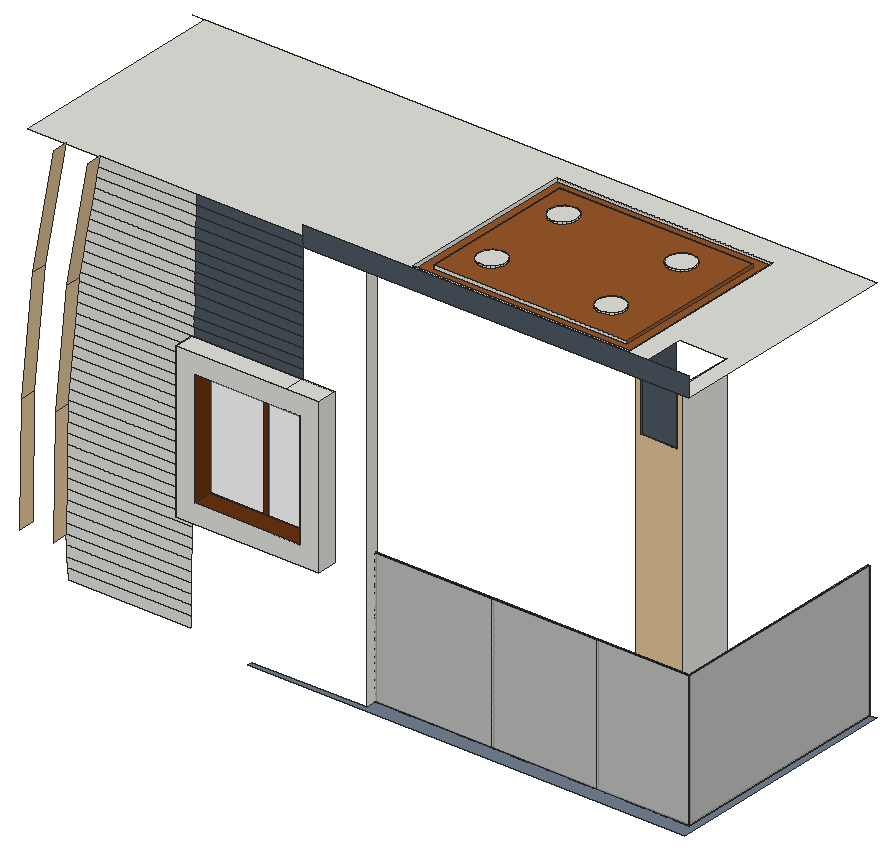
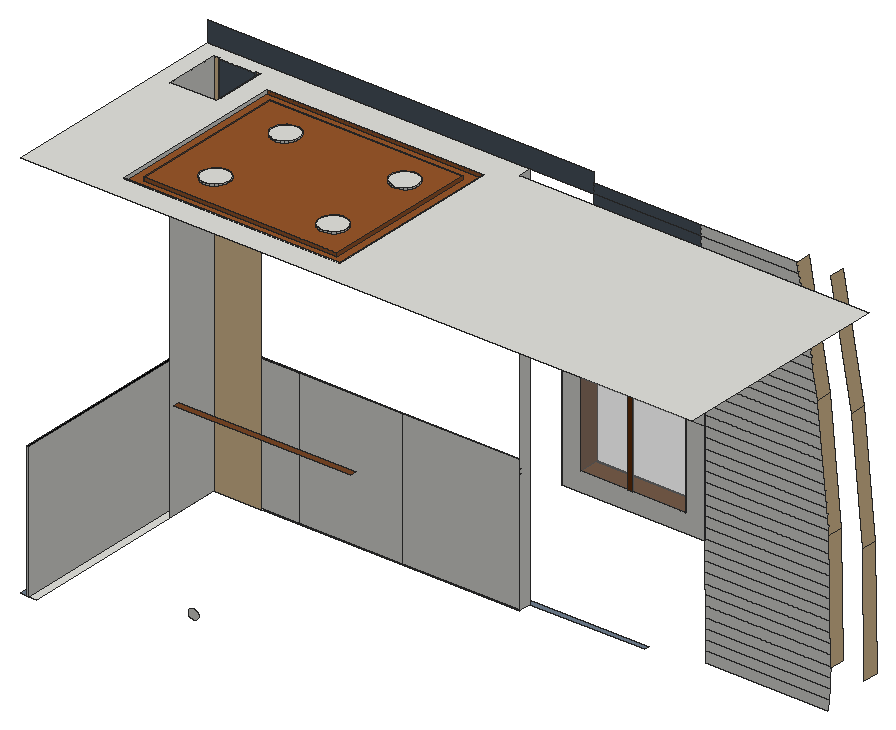
# SketchUp Ruby script. Lengths in inches.
U = 1.inch
M = Sketchup.active_model
def pt(a) = Geom::Point3d.new(a.map { |v| v * U })
def face(e, loops, mat)
  f = e.add_face(loops[0].map { |a| pt(a) })
  loops[1..].each { |l| e.add_face(l.map { |a| pt(a) }).erase! }
  f.material = f.back_material = mat if mat
  f
end
# faces: each face lists its corners as indices into pts; further lists are holes
def faces(e, pts, list, mat = nil) = list.each { |f| face(e, (f[0].is_a?(Array) ? f : [f]).map { |l| l.map { |i| pts[i] } }, mat) }
# xy, xz, yz: faces in a plane at the given z, y or x. An outline is a flat list of corners, or four numbers for a rectangle; further outlines are holes
def ring(l) = l.size == 4 ? [[l[0], l[1]], [l[2], l[1]], [l[2], l[3]], [l[0], l[3]]] : l.each_slice(2).to_a
def flat(e, list, mat, &to3) = list.each { |f| face(e, (f[0].is_a?(Array) ? f : [f]).map { |l| ring(l).map { |u, v| to3.(u, v) } }, mat) }
def xy(e, z, list, mat = nil) = flat(e, list, mat) { |x, y| [x, y, z] }
def xz(e, y, list, mat = nil) = flat(e, list, mat) { |x, z| [x, y, z] }
def yz(e, x, list, mat = nil) = flat(e, list, mat) { |y, z| [x, y, z] }
def lines(e, pts, list) = list.each { |a, b| e.add_line(pt(pts[a]), pt(pts[b])) }
# prism: a flat outline (further loops are holes) pulled along v
def prism(e, loops, v, mat = nil)
  f = face(e, loops, mat); d = Geom::Vector3d.new(v.map { |x| x * U })
  f.pushpull(f.normal.samedirection?(d) ? d.length : -d.length)
end
def box(e, o, s, mat = nil) = prism(e, [[o, [o[0] + s[0], o[1], o[2]], [o[0] + s[0], o[1] + s[1], o[2]], [o[0], o[1] + s[1], o[2]]]], [0, 0, s[2]], mat)
def at(x, y, z, deg = 0) = Geom::Transformation.translation(pt([x, y, z])) * Geom::Transformation.rotation(ORIGIN, Z_AXIS, deg.degrees)
def axes(o, x, y, z) = Geom::Transformation.new([*x, 0, *y, 0, *z, 0, *pt(o).to_a, 1])
def part(name) = M.definitions.add(name)
# library, detail: a bought-in or finely detailed component or shape, given as its bounding box
def library(name, o, s) = part(name).tap { |d| box(d.entities, o, s) }
def detail(e, o, s) = box(e.add_group.entities, o, s)
def put(e, d, t, mat = nil) = e.add_instance(d, t).tap { |i| i.material = mat if mat }
def group(e, t, mat = nil) = e.add_group.tap { |g| g.transformation = t; g.material = mat if mat }.entities
root = M.entities
M.materials.add("[0033_NavajoWhite]").color = [226, 197, 153]
M.materials.add("[0043_SaddleBrown]").color = [104, 51, 14]
M.materials.add("[0111_SlateGray]").color = [77, 88, 99]
M.materials.add("[0111_SlateGray]1").color = [112, 128, 144]
M.materials.add("[0137_Black]").color = [0, 0, 0]
M.materials.add("[Translucent Glass Gray]").color = [193, 193, 193]
M.materials["[Translucent Glass Gray]"].alpha = 0.5
M.materials.add("[Translucent Resin Crush Gray]").color = [184, 184, 184]
M.materials["[Translucent Resin Crush Gray]"].alpha = 0.8
M.materials.add("[Wood Cherry Original]").color = [152, 86, 42]
M.materials.add("[Wood Veneer 01]").color = [120, 70, 37]
xy(root,1006.5625,[[648,136.125,1210.3,139.125],[1210.3,136.125,1212.3,136.125,1212.3,538.125,1208.3,538.125,1208.3,139.125,1210.3,139.125],[648,139.125,1208.3,139.125,1208.3,538.125,1195.125,538.125,1195.125,142.125,648,142.125]])
xy(root,1006.5625,[[444,109.125,1224,109.125,1224,538.125,1212.3,538.125,1212.3,136.125,648,136.125,648,118.125,444,118.125]],"[0111_SlateGray]1")
xy(root,1217.72,[[336.04,82.125,592.16,118.125]])
xy(root,1246.5625,[[648,136.125,858.37,139.125],[858.37,136.125,1045.72,139.125],[1045.72,136.125,1210.3,139.125],[1210.3,136.125,1212.3,136.125,1212.3,538.125,1208.3,538.125,1208.3,139.125,1210.3,139.125]],"[0137_Black]")
xy(root,1251.48,[[369.8,82.125,558.4,118.125]],"[0043_SaddleBrown]")
xy(root,1411.875,[[624,538.125,939.8125,550.125]],"[Wood Veneer 01]")
xy(root,1458.02,[[391.68,95.13,389.33,95.2,387.08,95.88,385.08,97.12,383.47,98.83,382.36,100.9,381.82,103.18,381.89,105.53,382.57,107.78,383.8,109.78,385.51,111.39,387.58,112.5,389.87,113.04,392.22,112.97,394.47,112.29,396.47,111.06,398.08,109.35,399.1875,107.28,399.73,104.99,399.66,102.64,398.98,100.39,397.74,98.39,396.03,96.78,393.96,95.67],[453.68,95.13,451.33,95.2,449.08,95.88,447.08,97.12,445.47,98.83,444.36,100.9,443.82,103.18,443.89,105.53,444.57,107.78,445.8,109.78,447.51,111.39,449.58,112.5,451.87,113.04,454.22,112.97,456.47,112.29,458.47,111.06,460.08,109.35,461.1875,107.28,461.73,104.99,461.66,102.64,460.98,100.39,459.74,98.39,458.03,96.78,455.96,95.67],[516.12,95.13,513.77,95.2,511.52,95.88,509.52,97.12,507.91,98.83,506.8,100.9,506.26,103.18,506.33,105.53,507,107.78,508.24,109.78,509.95,111.39,512.02,112.5,514.31,113.04,516.66,112.97,518.91,112.29,520.9,111.06,522.51,109.35,523.625,107.28,524.17,104.99,524.09,102.64,523.42,100.39,522.18,98.39,520.47,96.78,518.4,95.67]])
xy(root,1458.02,[[[369.8,82.125,558.4,118.125],[391.68,95.13,393.96,95.67,396.03,96.78,397.74,98.39,398.98,100.39,399.66,102.64,399.73,104.99,399.1875,107.28,398.08,109.35,396.47,111.06,394.47,112.29,392.22,112.97,389.87,113.04,387.58,112.5,385.51,111.39,383.8,109.78,382.57,107.78,381.89,105.53,381.82,103.18,382.36,100.9,383.47,98.83,385.08,97.12,387.08,95.88,389.33,95.2],[453.68,95.13,455.96,95.67,458.03,96.78,459.74,98.39,460.98,100.39,461.66,102.64,461.73,104.99,461.1875,107.28,460.08,109.35,458.47,111.06,456.47,112.29,454.22,112.97,451.87,113.04,449.58,112.5,447.51,111.39,445.8,109.78,444.57,107.78,443.89,105.53,443.82,103.18,444.36,100.9,445.47,98.83,447.08,97.12,449.08,95.88,451.33,95.2],[516.12,95.13,518.4,95.67,520.47,96.78,522.18,98.39,523.42,100.39,524.09,102.64,524.17,104.99,523.625,107.28,522.51,109.35,520.9,111.06,518.91,112.29,516.66,112.97,514.31,113.04,512.02,112.5,509.95,111.39,508.24,109.78,507,107.78,506.33,105.53,506.26,103.18,506.8,100.9,507.91,98.83,509.52,97.12,511.52,95.88,513.77,95.2]]],"[0043_SaddleBrown]")
xy(root,1491.78,[[336.04,82.125,534.32,118.125],[534.32,82.125,592.16,118.125]])
xy(root,1596.63,[[1110.4375,146.89,1112.4375,229.71]],"[0111_SlateGray]")
xy(root,1598.625,[[1119.45,142.125,1184.58,144.125]],"[0111_SlateGray]")
xy(root,1698,[[[688.77,171.82,1075.45,493.51],[709.36,192.42,1054.86,472.91]]],"[Wood Cherry Original]")
xy(root,1704,[[[648,118.125,648,142.125,24,142.125,24,538.125,1224,538.125,1224,118.125],[688.77,171.82,1075.45,493.51],[1110.4375,142.125,1119.45,142.125,1119.45,144.125,1184.58,144.125,1184.58,142.125,1195.125,142.125,1195.125,239.75,1110.4375,239.75,1110.4375,229.71,1112.4375,229.71,1112.4375,146.89,1110.4375,146.89]]])
xy(root,1704,[[[709.36,192.42,1054.86,472.91],[765.56,231.1,771.66,232.53,777.18,235.49,781.75,239.78,785.05,245.1,786.86,251.1,787.0625,257.36,785.63,263.46,782.67,268.99,778.39,273.55,773.0625,276.86,767.0625,278.67,760.8,278.87,754.7,277.4375,749.18,274.48,744.61,270.19,741.31,264.87,739.5,258.87,739.3,252.61,740.73,246.51,743.6875,240.99,747.97,236.42,753.3,233.11,759.29,231.3],[978.37,231.1,984.47,232.53,989.99,235.49,994.56,239.78,997.86,245.1,999.68,251.1,999.875,257.36,998.44,263.46,995.49,268.99,991.2,273.55,985.875,276.86,979.875,278.67,973.61,278.87,967.51,277.4375,961.99,274.48,957.42,270.19,954.12,264.87,952.31,258.87,952.11,252.61,953.54,246.51,956.5,240.99,960.79,236.42,966.11,233.11,972.11,231.3],[978.37,388.48,984.47,389.91,989.99,392.87,994.56,397.15,997.86,402.48,999.68,408.48,999.875,414.74,998.44,420.84,995.49,426.36,991.2,430.93,985.875,434.23,979.875,436.04,973.61,436.24,967.51,434.8125,961.99,431.85,957.42,427.57,954.12,422.24,952.31,416.25,952.11,409.98,953.54,403.88,956.5,398.36,960.79,393.79,966.11,390.49,972.11,388.68],[765.56,391.23,771.66,392.66,777.18,395.62,781.75,399.9,785.05,405.23,786.86,411.23,787.0625,417.49,785.63,423.59,782.67,429.11,778.39,433.68,773.0625,436.98,767.0625,438.79,760.8,438.99,754.7,437.5625,749.18,434.6,744.61,430.32,741.31,424.99,739.5,419,739.3,412.73,740.73,406.63,743.6875,401.11,747.97,396.54,753.3,393.24,759.29,391.43]]],"[Wood Cherry Original]")
xy(root,1707,[[765.56,231.1,759.29,231.3,753.3,233.11,747.97,236.42,743.6875,240.99,740.73,246.51,739.3,252.61,739.5,258.87,741.31,264.87,744.61,270.19,749.18,274.48,754.7,277.4375,760.8,278.87,767.0625,278.67,773.0625,276.86,778.39,273.55,782.67,268.99,785.63,263.46,787.0625,257.36,786.86,251.1,785.05,245.1,781.75,239.78,777.18,235.49,771.66,232.53],[978.37,231.1,972.11,231.3,966.11,233.11,960.79,236.42,956.5,240.99,953.54,246.51,952.11,252.61,952.31,258.87,954.12,264.87,957.42,270.19,961.99,274.48,967.51,277.4375,973.61,278.87,979.875,278.67,985.875,276.86,991.2,273.55,995.49,268.99,998.44,263.46,999.875,257.36,999.68,251.1,997.86,245.1,994.56,239.78,989.99,235.49,984.47,232.53],[978.37,388.48,972.11,388.68,966.11,390.49,960.79,393.79,956.5,398.36,953.54,403.88,952.11,409.98,952.31,416.25,954.12,422.24,957.42,427.57,961.99,431.85,967.51,434.8125,973.61,436.24,979.875,436.04,985.875,434.23,991.2,430.93,995.49,426.36,998.44,420.84,999.875,414.74,999.68,408.48,997.86,402.48,994.56,397.15,989.99,392.87,984.47,389.91],[765.56,391.23,759.29,391.43,753.3,393.24,747.97,396.54,743.6875,401.11,740.73,406.63,739.3,412.73,739.5,419,741.31,424.99,744.61,430.32,749.18,434.6,754.7,437.5625,760.8,438.99,767.0625,438.79,773.0625,436.98,778.39,433.68,782.67,429.11,785.63,423.59,787.0625,417.49,786.86,411.23,785.05,405.23,781.75,399.9,777.18,395.62,771.66,392.66]])
xz(root,82.125,[[[336.04,1217.72,592.16,1491.78],[369.8,1251.48,558.4,1458.02]]])
xz(root,118.125,[[115.22,1023.78,333.42,1023.78,333.66,1041.78,114.0625,1041.78],[114.0625,1041.78,333.66,1041.78,333.91,1059.78,112.9,1059.78],[112.9,1059.78,333.91,1059.78,334.15,1077.78,111.74,1077.78],[111.74,1077.78,334.15,1077.78,334.39,1095.78,110.79,1095.78,110.76,1093.03],[110.79,1095.78,334.39,1095.78,334.63,1113.78,111.04,1113.78],
  [111.04,1113.78,334.63,1113.78,334.88,1131.78,111.28,1131.78],[111.28,1131.78,334.88,1131.78,335.12,1149.78,111.52,1149.78],[111.52,1149.78,335.12,1149.78,335.36,1167.78,111.77,1167.78],[111.77,1167.78,335.36,1167.78,335.61,1185.78,112.01,1185.78],[112.01,1185.78,335.61,1185.78,335.85,1203.78,112.25,1203.78],
  [112.25,1203.78,335.85,1203.78,336.04,1217.72,336.04,1221.78,112.49,1221.78],[[336.04,1217.72,592.16,1491.78],[369.8,1251.48,558.4,1458.02]],[112.49,1221.78,336.04,1221.78,336.04,1239.78,112.74,1239.78],[112.74,1239.78,336.04,1239.78,336.04,1257.78,112.98,1257.78],[112.98,1257.78,336.04,1257.78,336.04,1275.78,113.22,1275.78],
  [113.22,1275.78,336.04,1275.78,336.04,1293.78,113.47,1293.78],[113.47,1293.78,336.04,1293.78,336.04,1311.78,114.36,1311.78,113.6,1303.95],[114.36,1311.78,336.04,1311.78,336.04,1329.78,116.09,1329.78],[116.09,1329.78,336.04,1329.78,336.04,1347.78,117.83,1347.78],[117.83,1347.78,336.04,1347.78,336.04,1365.78,119.56,1365.78],
  [119.56,1365.78,336.04,1365.78,336.04,1383.78,121.29,1383.78],[121.29,1383.78,336.04,1383.78,336.04,1401.78,123.03,1401.78],[123.03,1401.78,336.04,1401.78,336.04,1419.78,124.76,1419.78],[124.76,1419.78,336.04,1419.78,336.04,1437.78,126.49,1437.78],[126.49,1437.78,336.04,1437.78,336.04,1455.78,128.23,1455.78],
  [128.23,1455.78,336.04,1455.78,336.04,1473.78,129.96,1473.78],[129.96,1473.78,336.04,1473.78,336.04,1491.78,131.7,1491.78],[131.7,1491.78,339.74,1491.78,339.96,1507.89,133.25,1507.89],[133.25,1507.89,339.96,1507.89,340.17,1524,135.65,1524,133.83,1513.92],[135.65,1524,340.17,1524,340.42,1542,138.9,1542],
  [138.9,1542,340.42,1542,340.66,1560,142.14,1560],[142.14,1560,340.66,1560,340.9,1578,145.39,1578],[145.39,1578,340.9,1578,341.15,1596,148.64,1596],[148.64,1596,341.15,1596,341.39,1614,151.89,1614],[151.89,1614,341.39,1614,341.63,1632,155.14,1632],
  [155.14,1632,341.63,1632,341.875,1650,158.39,1650],[158.39,1650,341.875,1650,342.12,1668,161.64,1668],[161.64,1668,342.12,1668,342.36,1686,164.88,1686],[164.88,1686,342.36,1686,342.6,1704,168.13,1704],[168.13,1704,342.6,1704,342.85,1722,171.42,1722,171.29,1721.51]])
xz(root,118.125,[[464.1,1251.48,473.1,1458.02]],"[0043_SaddleBrown]")
xz(root,118.125,[[339.74,1491.78,534.32,1491.78,534.32,1507.89,339.96,1507.89],[339.96,1507.89,534.32,1507.89,534.32,1524,340.17,1524],[340.17,1524,534.32,1524,534.32,1542,340.42,1542],[340.42,1542,534.32,1542,534.32,1560,340.66,1560],[340.66,1560,534.32,1560,534.32,1578,340.9,1578],
  [340.9,1578,534.32,1578,534.32,1596,341.15,1596],[341.15,1596,534.32,1596,534.32,1614,341.39,1614],[341.39,1614,534.32,1614,534.32,1632,341.63,1632],[341.63,1632,534.32,1632,534.32,1650,341.875,1650],[341.875,1650,534.32,1650,534.32,1668,342.12,1668],
  [342.12,1668,534.32,1668,534.32,1686,342.36,1686],[342.36,1686,534.32,1686,534.32,1704,342.6,1704],[342.6,1704,534.32,1704,534.32,1722,342.85,1722],[534.32,1704,1224,1740]],"[0111_SlateGray]")
xz(root,118.125,[[369.8,1251.48,464.1,1458.02],[473.1,1251.48,558.4,1458.02]],"[Translucent Glass Gray]")
xz(root,136.125,[[1210.3,1006.5625,1212.3,1246.5625]],"[0137_Black]")
xz(root,136.125,[[648,1006.5625,858.37,1246.5625],[858.37,1006.5625,1045.72,1246.5625],[1045.72,1006.5625,1210.3,1246.5625]],"[Translucent Resin Crush Gray]")
xz(root,139.125,[[648,1006.5625,858.37,1246.5625],[858.37,1006.5625,1045.72,1246.5625],[1045.72,1006.5625,1208.3,1246.5625],[1208.3,1006.5625,1210.3,1246.5625]])
xz(root,142.125,[[1110.4375,1006.5625,1195.125,1006.5625,1195.125,1704,1184.58,1704,1184.58,1598.625,1119.45,1598.625,1119.45,1704,1110.4375,1704]],"[0033_NavajoWhite]")
xz(root,144.125,[[1119.45,1598.625,1184.58,1704]],"[0111_SlateGray]")
xz(root,146.89,[[1110.4375,1596.63,1112.4375,1704]])
xz(root,171.82,[[688.77,1698,1075.45,1704]],"[Wood Cherry Original]")
xz(root,192.42,[[709.36,1698,1054.86,1704]])
xz(root,229.71,[[1110.4375,1596.63,1112.4375,1704]],"[0111_SlateGray]")
xz(root,472.91,[[709.36,1698,1054.86,1704]],"[Wood Cherry Original]")
xz(root,493.51,[[688.77,1698,1075.45,1704]])
xz(root,538.125,[[1208.3,1006.5625,1212.3,1246.5625]])
xz(root,550.125,[[904.46,1081.11,906.79,1081.41,908.96,1082.3125,910.82,1083.74,912.25,1085.61,913.15,1087.78,913.46,1090.11,913.15,1092.44,912.25,1094.61,910.82,1096.47,908.96,1097.9,906.79,1098.8,904.46,1099.11,902.13,1098.8,899.96,1097.9,898.09,1096.47,896.66,1094.61,895.77,1092.44,895.46,1090.11,895.77,1087.78,896.66,1085.61,898.09,1083.74,899.96,1082.3125,902.13,1081.41]])
yz(root,336.04,[[82.125,1217.72,118.125,1491.78]])
yz(root,369.8,[[82.125,1251.48,118.125,1458.02]],"[0043_SaddleBrown]")
yz(root,558.4,[[82.125,1251.48,118.125,1458.02]],"[0043_SaddleBrown]")
yz(root,592.16,[[82.125,1217.72,118.125,1491.78]])
yz(root,648,[[118.125,1006.5625,136.125,1006.5625,136.125,1246.5625,139.125,1246.5625,139.125,1006.5625,142.125,1006.5625,142.125,1704,118.125,1704],[136.125,1006.5625,139.125,1246.5625]])
yz(root,688.77,[[171.82,1698,493.51,1704]])
yz(root,709.36,[[192.42,1698,472.91,1704]],"[Wood Cherry Original]")
yz(root,1054.86,[[192.42,1698,472.91,1704]],"[Wood Cherry Original]")
yz(root,1075.45,[[171.82,1698,493.51,1704]])
yz(root,1112.4375,[[146.89,1596.63,229.71,1704]],"[0111_SlateGray]")
yz(root,1119.45,[[142.125,1598.625,144.125,1704]],"[0111_SlateGray]")
yz(root,1184.58,[[142.125,1598.625,144.125,1704]],"[0111_SlateGray]")
yz(root,1195.125,[[142.125,1006.5625,239.75,1704]])
yz(root,1208.3,[[139.125,1006.5625,538.125,1246.5625]])
yz(root,1210.3,[[136.125,1006.5625,139.125,1246.5625]])
yz(root,1212.3,[[136.125,1006.5625,538.125,1246.5625]],"[Translucent Resin Crush Gray]")
p = [[53.6,118.125,1303.95],[50.76,118.125,1093.03],[50.76,91.125,1093.03],[53.6,91.125,1303.95],[113.47,118.125,1293.78],[113.6,118.125,1303.95],
  [113.6,91.125,1303.95],[110.76,91.125,1093.03],[110.76,118.125,1093.03],[110.79,118.125,1095.78],[111.04,118.125,1113.78],[111.28,118.125,1131.78],
  [111.52,118.125,1149.78],[111.77,118.125,1167.78],[112.01,118.125,1185.78],[112.25,118.125,1203.78],[112.49,118.125,1221.78],[112.74,118.125,1239.78],
  [112.98,118.125,1257.78],[113.22,118.125,1275.78],[73.83,118.125,1513.92],[73.83,91.125,1513.92],[133.25,118.125,1507.89],[133.83,118.125,1513.92],
  [133.83,91.125,1513.92],[114.36,118.125,1311.78],[116.09,118.125,1329.78],[117.83,118.125,1347.78],[119.56,118.125,1365.78],[121.29,118.125,1383.78],
  [123.03,118.125,1401.78],[124.76,118.125,1419.78],[126.49,118.125,1437.78],[128.23,118.125,1455.78],[129.96,118.125,1473.78],[131.7,118.125,1491.78],
  [111.29,118.125,1721.51],[111.29,91.125,1721.51],[168.13,118.125,1704],[171.29,118.125,1721.51],[171.29,91.125,1721.51],[135.65,118.125,1524],
  [138.9,118.125,1542],[142.14,118.125,1560],[145.39,118.125,1578],[148.64,118.125,1596],[151.89,118.125,1614],[155.14,118.125,1632],
  [158.39,118.125,1650],[161.64,118.125,1668],[164.88,118.125,1686],[765.56,231.1,1704],[759.29,231.3,1704],[759.29,231.3,1707],
  [765.56,231.1,1707],[771.66,232.53,1704],[771.66,232.53,1707],[978.37,231.1,1704],[972.11,231.3,1704],[972.11,231.3,1707],
  [978.37,231.1,1707],[984.47,232.53,1704],[984.47,232.53,1707],[753.3,233.11,1704],[753.3,233.11,1707],[966.11,233.11,1704],
  [966.11,233.11,1707],[777.18,235.49,1704],[777.18,235.49,1707],[989.99,235.49,1704],[989.99,235.49,1707],[747.97,236.42,1704],
  [747.97,236.42,1707],[960.79,236.42,1704],[960.79,236.42,1707],[781.75,239.78,1704],[781.75,239.78,1707],[994.56,239.78,1704],
  [994.56,239.78,1707],[743.6875,240.99,1704],[743.6875,240.99,1707],[956.5,240.99,1704],[956.5,240.99,1707],[785.05,245.1,1704],
  [785.05,245.1,1707],[997.86,245.1,1704],[997.86,245.1,1707],[740.73,246.51,1704],[740.73,246.51,1707],[953.54,246.51,1704],
  [953.54,246.51,1707],[786.86,251.1,1704],[786.86,251.1,1707],[999.68,251.1,1704],[999.68,251.1,1707],[739.3,252.61,1704],
  [739.3,252.61,1707],[952.11,252.61,1704],[952.11,252.61,1707],[787.0625,257.36,1704],[787.0625,257.36,1707],[999.875,257.36,1704],
  [999.875,257.36,1707],[739.5,258.87,1704],[739.5,258.87,1707],[952.31,258.87,1704],[952.31,258.87,1707],[785.63,263.46,1704],
  [785.63,263.46,1707],[998.44,263.46,1704],[998.44,263.46,1707],[741.31,264.87,1704],[741.31,264.87,1707],[954.12,264.87,1704],
  [954.12,264.87,1707],[782.67,268.99,1704],[782.67,268.99,1707],[995.49,268.99,1704],[995.49,268.99,1707],[744.61,270.19,1704],
  [744.61,270.19,1707],[957.42,270.19,1704],[957.42,270.19,1707],[778.39,273.55,1704],[778.39,273.55,1707],[991.2,273.55,1704],
  [991.2,273.55,1707],[749.18,274.48,1704],[749.18,274.48,1707],[961.99,274.48,1704],[961.99,274.48,1707],[773.0625,276.86,1704],
  [773.0625,276.86,1707],[985.875,276.86,1704],[985.875,276.86,1707],[754.7,277.4375,1704],[754.7,277.4375,1707],[967.51,277.4375,1704],
  [967.51,277.4375,1707],[767.0625,278.67,1704],[767.0625,278.67,1707],[979.875,278.67,1704],[979.875,278.67,1707],[760.8,278.87,1704],
  [760.8,278.87,1707],[973.61,278.87,1704],[973.61,278.87,1707],[978.37,388.48,1704],[972.11,388.68,1704],[972.11,388.68,1707],
  [978.37,388.48,1707],[984.47,389.91,1704],[984.47,389.91,1707],[966.11,390.49,1704],[966.11,390.49,1707],[989.99,392.87,1704],
  [989.99,392.87,1707],[960.79,393.79,1704],[960.79,393.79,1707],[765.56,391.23,1704],[759.29,391.43,1704],[759.29,391.43,1707],
  [765.56,391.23,1707],[771.66,392.66,1704],[771.66,392.66,1707],[753.3,393.24,1704],[753.3,393.24,1707],[777.18,395.62,1704],
  [777.18,395.62,1707],[994.56,397.15,1704],[994.56,397.15,1707],[747.97,396.54,1704],[747.97,396.54,1707],[956.5,398.36,1704],
  [956.5,398.36,1707],[781.75,399.9,1704],[781.75,399.9,1707],[743.6875,401.11,1704],[743.6875,401.11,1707],[997.86,402.48,1704],
  [997.86,402.48,1707],[953.54,403.88,1704],[953.54,403.88,1707],[785.05,405.23,1704],[785.05,405.23,1707],[740.73,406.63,1704],
  [740.73,406.63,1707],[999.68,408.48,1704],[999.68,408.48,1707],[952.11,409.98,1704],[952.11,409.98,1707],[786.86,411.23,1704],
  [786.86,411.23,1707],[739.3,412.73,1704],[739.3,412.73,1707],[999.875,414.74,1704],[999.875,414.74,1707],[952.31,416.25,1704],
  [952.31,416.25,1707],[787.0625,417.49,1704],[787.0625,417.49,1707],[739.5,419,1704],[739.5,419,1707],[998.44,420.84,1704],
  [998.44,420.84,1707],[954.12,422.24,1704],[954.12,422.24,1707],[785.63,423.59,1704],[785.63,423.59,1707],[741.31,424.99,1704],
  [741.31,424.99,1707],[995.49,426.36,1704],[995.49,426.36,1707],[957.42,427.57,1704],[957.42,427.57,1707],[782.67,429.11,1704],
  [782.67,429.11,1707],[744.61,430.32,1704],[744.61,430.32,1707],[991.2,430.93,1704],[991.2,430.93,1707],[961.99,431.85,1704],
  [961.99,431.85,1707],[778.39,433.68,1704],[778.39,433.68,1707],[749.18,434.6,1704],[749.18,434.6,1707],[985.875,434.23,1704],
  [985.875,434.23,1707],[967.51,434.8125,1704],[967.51,434.8125,1707],[773.0625,436.98,1704],[773.0625,436.98,1707],[979.875,436.04,1704],
  [979.875,436.04,1707],[754.7,437.5625,1704],[754.7,437.5625,1707],[973.61,436.24,1704],[973.61,436.24,1707],[767.0625,438.79,1704],
  [767.0625,438.79,1707],[760.8,438.99,1704],[760.8,438.99,1707],[24,538.125,1704],[0,538.125,1704]]
faces(root,p,[[0,1,2,3],[4,5,6,7,8,9,10,11,12,13,14,15,16,17,18,19],[20,0,3,21],[22,23,24,6,5,25,26,27,28,29,30,31,32,33,34,35],[36,20,21,37],[38,39,40,24,23,41,42,43,44,45,46,47,48,49,50]],"[0033_NavajoWhite]")
faces(root,p,[[51,52,53,54],[55,51,54,56],[57,58,59,60],[61,57,60,62],[52,63,64,53],[58,65,66,59],[67,55,56,68],[69,61,62,70],
  [63,71,72,64],[65,73,74,66],[75,67,68,76],[77,69,70,78],[71,79,80,72],[73,81,82,74],[83,75,76,84],[85,77,78,86],
  [79,87,88,80],[81,89,90,82],[91,83,84,92],[93,85,86,94],[87,95,96,88],[89,97,98,90],[99,91,92,100],[101,93,94,102],
  [95,103,104,96],[97,105,106,98],[107,99,100,108],[109,101,102,110],[103,111,112,104],[105,113,114,106],[115,107,108,116],[117,109,110,118],
  [111,119,120,112],[113,121,122,114],[123,115,116,124],[125,117,118,126],[119,127,128,120],[121,129,130,122],[131,123,124,132],[133,125,126,134],
  [127,135,136,128],[129,137,138,130],[139,131,132,140],[141,133,134,142],[135,143,144,136],[137,145,146,138],[143,139,140,144],[145,141,142,146],
  [147,148,149,150],[151,147,150,152],[148,153,154,149],[155,151,152,156],[153,157,158,154],[159,160,161,162],[163,159,162,164],[160,165,166,161],
  [167,163,164,168],[169,155,156,170],[165,171,172,166],[157,173,174,158],[175,167,168,176],[171,177,178,172],[179,169,170,180],[173,181,182,174],
  [183,175,176,184],[177,185,186,178],[187,179,180,188],[181,189,190,182],[191,183,184,192],[185,193,194,186],[195,187,188,196],[189,197,198,190],
  [199,191,192,200],[193,201,202,194],[203,195,196,204],[197,205,206,198],[207,199,200,208],[201,209,210,202],[211,203,204,212],[205,213,214,206],
  [215,207,208,216],[209,217,218,210],[219,211,212,220],[213,221,222,214],[223,215,216,224],[217,225,226,218],[227,219,220,228],[221,229,230,222],
  [231,223,224,232],[233,227,228,234],[225,235,236,226],[229,237,238,230],[237,233,234,238],[239,231,232,240],[235,241,242,236],[241,239,240,242]])
lines(root,p,[[243,244]])
